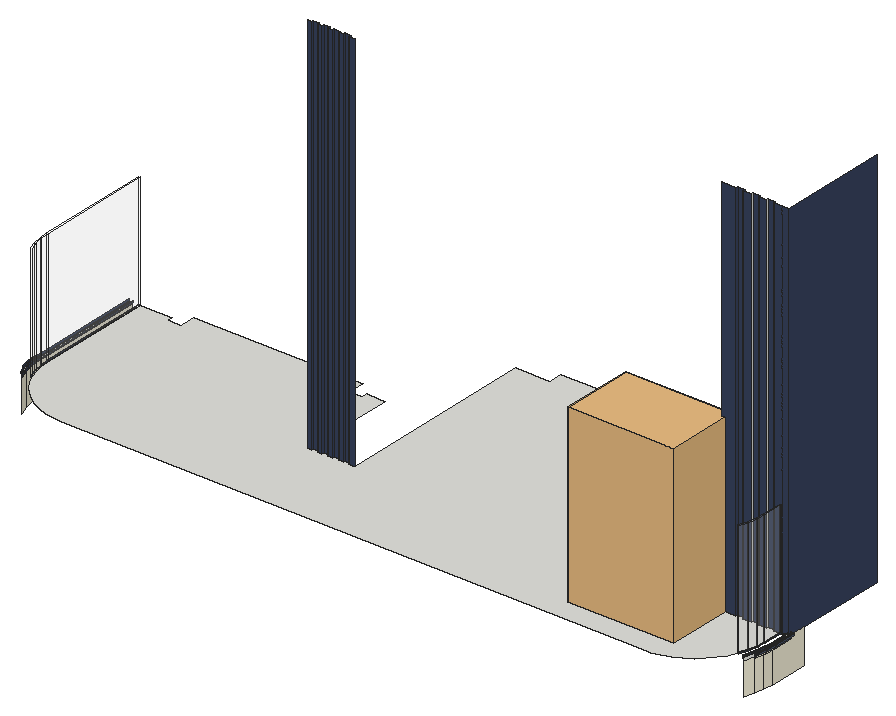
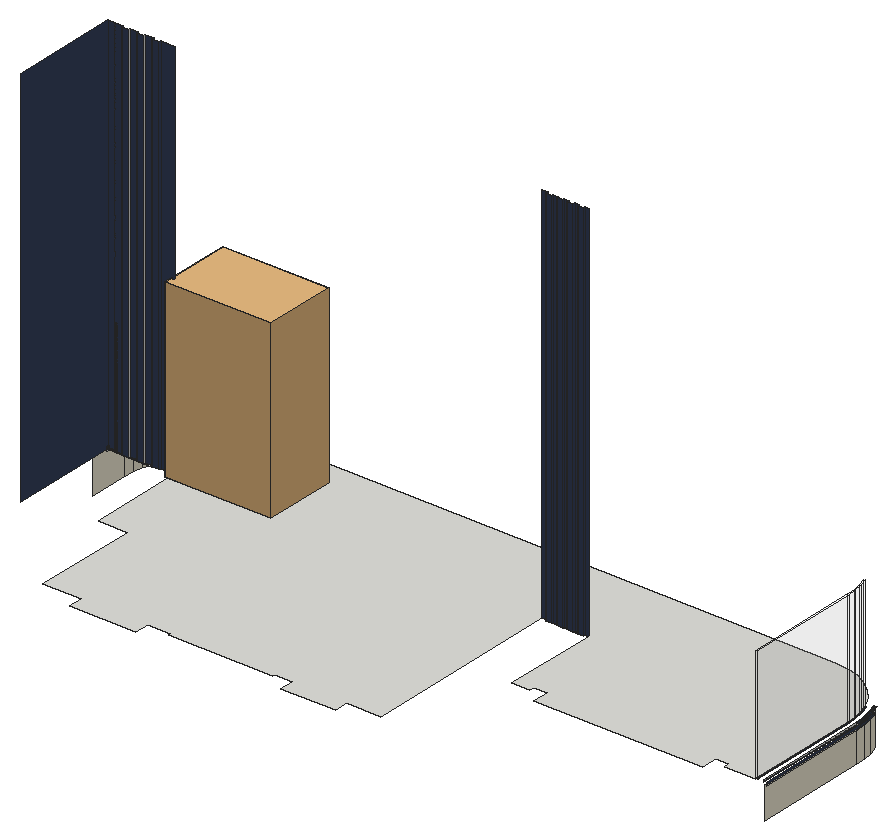
# SketchUp Ruby script. Lengths in inches.
U = 1.inch
M = Sketchup.active_model
def pt(a) = Geom::Point3d.new(a.map { |v| v * U })
def face(e, loops, mat)
  f = e.add_face(loops[0].map { |a| pt(a) })
  loops[1..].each { |l| e.add_face(l.map { |a| pt(a) }).erase! }
  f.material = f.back_material = mat if mat
  f
end
# faces: each face lists its corners as indices into pts; further lists are holes
def faces(e, pts, list, mat = nil) = list.each { |f| face(e, (f[0].is_a?(Array) ? f : [f]).map { |l| l.map { |i| pts[i] } }, mat) }
# xy, xz, yz: faces in a plane at the given z, y or x. An outline is a flat list of corners, or four numbers for a rectangle; further outlines are holes
def ring(l) = l.size == 4 ? [[l[0], l[1]], [l[2], l[1]], [l[2], l[3]], [l[0], l[3]]] : l.each_slice(2).to_a
def flat(e, list, mat, &to3) = list.each { |f| face(e, (f[0].is_a?(Array) ? f : [f]).map { |l| ring(l).map { |u, v| to3.(u, v) } }, mat) }
def xy(e, z, list, mat = nil) = flat(e, list, mat) { |x, y| [x, y, z] }
def xz(e, y, list, mat = nil) = flat(e, list, mat) { |x, z| [x, y, z] }
def yz(e, x, list, mat = nil) = flat(e, list, mat) { |y, z| [x, y, z] }
def lines(e, pts, list) = list.each { |a, b| e.add_line(pt(pts[a]), pt(pts[b])) }
# prism: a flat outline (further loops are holes) pulled along v
def prism(e, loops, v, mat = nil)
  f = face(e, loops, mat); d = Geom::Vector3d.new(v.map { |x| x * U })
  f.pushpull(f.normal.samedirection?(d) ? d.length : -d.length)
end
def box(e, o, s, mat = nil) = prism(e, [[o, [o[0] + s[0], o[1], o[2]], [o[0] + s[0], o[1] + s[1], o[2]], [o[0], o[1] + s[1], o[2]]]], [0, 0, s[2]], mat)
def at(x, y, z, deg = 0) = Geom::Transformation.translation(pt([x, y, z])) * Geom::Transformation.rotation(ORIGIN, Z_AXIS, deg.degrees)
def axes(o, x, y, z) = Geom::Transformation.new([*x, 0, *y, 0, *z, 0, *pt(o).to_a, 1])
def part(name) = M.definitions.add(name)
# library, detail: a bought-in or finely detailed component or shape, given as its bounding box
def library(name, o, s) = part(name).tap { |d| box(d.entities, o, s) }
def detail(e, o, s) = box(e.add_group.entities, o, s)
def put(e, d, t, mat = nil) = e.add_instance(d, t).tap { |i| i.material = mat if mat }
def group(e, t, mat = nil) = e.add_group.tap { |g| g.transformation = t; g.material = mat if mat }.entities
root = M.entities
M.materials.add("0344 AP 9635 Ganges Midnight-N").color = [69, 80, 105]
M.materials.add("0360 AP 9644 Monsoon Midnight-N").color = [56, 67, 95]
M.materials.add("0905 AP 7844 MILD YELLOW").color = [242, 237, 215]
M.materials.add("Glass Clear 001").color = [246, 246, 246]
M.materials["Glass Clear 001"].alpha = 0.1
c1 = library("Ficus triangularis Variegata 002",[-17,-11.8,0.01],[33.04,22.7,54.61])
xy(root,132,[[57,32.69,238.5625,32.69,241.34,32.87,244.0625,33.41,246.69,34.31,249.1875,35.54,251.5,37.08,253.59,38.91,255.42,41,256.96,43.3125,258.19,45.81,259.09,48.4375,259.63,51.16,259.81,53.9375,259.81,60.0625,257.875,60.0625,257.875,60.55,255.6875,60.55,255.6875,60.0625,253.125,60.0625,253.125,60.55,250.9375,60.55,250.9375,60.0625,248.375,60.0625,248.375,60.55,246.1875,60.55,246.1875,60.0625,241.5625,60.0625,241.5625,89.9375,232.5625,89.9375,232.5625,122.9375,220.5625,122.9375,220.5625,127.4375,199.92,127.4375,199.92,122.9375,192.74,122.9375,192.74,123.43,160.18,123.43,160.18,122.9375,154.56,122.9375,154.56,127.4375,137.54,127.4375,137.54,122.9375,126.8125,122.9375,126.8125,60.0625,125.0625,60.0625,125.0625,60.55,123.25,60.55,123.25,60.0625,121.75,60.0625,121.75,60.55,119.9375,60.55,119.9375,60.0625,118.4375,60.0625,118.4375,60.55,116.625,60.55,116.625,60.0625,115.125,60.0625,115.125,60.55,113.3125,60.55,113.3125,60.0625,112.1875,60.0625,112.1875,89.9375,106.59,89.9375,106.59,88.375,102.41,88.375,102.41,93.58,49.72,93.58,49.72,88.375,45.54,88.375,45.54,89.9375,35.75,89.9375,35.75,53.9375,35.94,51.16,36.48,48.4375,37.37,45.81,38.6,43.3125,40.14,41,41.98,38.91,44.07,37.08,46.375,35.54,48.87,34.31,51.5,33.41,54.23,32.87],[115.125,60.0625,116.625,60.55],[118.4375,60.0625,119.9375,60.55],[121.75,60.0625,123.25,60.55],[248.375,60.0625,250.9375,60.55],
  [253.125,60.0625,255.6875,60.55],[257.875,60.0625,262.21,60.55],[262.21,60.0625,262.5625,60.55],[262.21,60.55,262.5625,60.91]])
xz(root,60.0625,[[259.81,132,260.1875,168],[262.21,132,262.5625,132.625]])
xz(root,60.0625,[[112.1875,132,113.3125,252],[115.125,132,116.625,252],[118.4375,132,119.9375,252],[121.75,132,123.25,252],[125.0625,132,126.8125,252],
  [241.5625,132,246.1875,252],[248.375,132,250.9375,252],[253.125,132,255.6875,252],[257.875,132,259.81,132,259.81,168.3125,260.1875,168.3125,260.1875,132.1875,260.4375,132.1875,260.4375,252,257.875,252],[260.1875,132,260.4375,132.1875],
  [260.4375,132,262.21,132.1875],[262.5625,132,262.625,252],[260.4375,132.1875,262.21,132.1875,262.21,132.8125,262.5625,132.8125,262.5625,252,260.4375,252],[262.21,132.625,262.5625,132.8125]],"0360 AP 9644 Monsoon Midnight-N")
xz(root,60.47,[[262.48,132.5625,262.5625,132.625]])
xz(root,60.47,[[262.48,132.625,262.5625,132.8125],[262.5625,132.625,262.97,132.8125]],"0360 AP 9644 Monsoon Midnight-N")
xz(root,60.55,[[262.5625,131.3125,263.05,132],[262.5625,132,263.05,132.625]])
xz(root,60.55,[[113.3125,132,115.125,252],[116.625,132,118.4375,252],[119.9375,132,121.75,252],[123.25,132,125.0625,252],[246.1875,132,248.375,252],
  [250.9375,132,253.125,252],[255.6875,132,257.875,252],[262.5625,132.625,263.05,132.8125]],"0360 AP 9644 Monsoon Midnight-N")
xz(root,60.91,[[262.5625,132,263.41,132.5625],[262.5625,132.5625,263.41,132.625]])
xz(root,60.91,[[262.5625,132.625,263.41,132.8125]],"0360 AP 9644 Monsoon Midnight-N")
xz(root,60.99,[[262.48,132.5625,263.49,132.625]])
xz(root,60.99,[[262.48,132.625,263.49,132.8125]],"0360 AP 9644 Monsoon Midnight-N")
yz(root,32.15,[[53.9375,132,89.9375,132.5625]],"0360 AP 9644 Monsoon Midnight-N")
yz(root,32.51,[[53.9375,131.3125,89.9375,132]],"0905 AP 7844 MILD YELLOW")
yz(root,33,[[53.9375,121.25,89.9375,131.3125]],"0905 AP 7844 MILD YELLOW")
yz(root,33.35,[[53.9375,132.1875,89.9375,132.625]])
yz(root,33.35,[[53.9375,132,89.9375,132.1875]],"0360 AP 9644 Monsoon Midnight-N")
yz(root,35.375,[[53.9375,132,89.9375,132.1875]],"0360 AP 9644 Monsoon Midnight-N")
yz(root,35.375,[[53.9375,132.1875,89.9375,168]],"Glass Clear 001")
yz(root,35.75,[[53.9375,132,89.9375,168]],"Glass Clear 001")
yz(root,113.3125,[[60.0625,132,60.55,252]],"0360 AP 9644 Monsoon Midnight-N")
yz(root,115.125,[[60.0625,132,60.55,252]],"0360 AP 9644 Monsoon Midnight-N")
yz(root,116.625,[[60.0625,132,60.55,252]],"0360 AP 9644 Monsoon Midnight-N")
yz(root,118.4375,[[60.0625,132,60.55,252]],"0360 AP 9644 Monsoon Midnight-N")
yz(root,119.9375,[[60.0625,132,60.55,252]],"0360 AP 9644 Monsoon Midnight-N")
yz(root,121.75,[[60.0625,132,60.55,252]],"0360 AP 9644 Monsoon Midnight-N")
yz(root,123.25,[[60.0625,132,60.55,252]],"0360 AP 9644 Monsoon Midnight-N")
yz(root,125.0625,[[60.0625,132,60.55,252]],"0360 AP 9644 Monsoon Midnight-N")
yz(root,246.1875,[[60.0625,132,60.55,252]],"0360 AP 9644 Monsoon Midnight-N")
yz(root,248.375,[[60.0625,132,60.55,252]],"0360 AP 9644 Monsoon Midnight-N")
yz(root,250.9375,[[60.0625,132,60.55,252]])
yz(root,253.125,[[60.0625,132,60.55,252]],"0360 AP 9644 Monsoon Midnight-N")
yz(root,255.6875,[[60.0625,132,60.55,252]])
yz(root,257.875,[[60.0625,132,60.55,252]],"0360 AP 9644 Monsoon Midnight-N")
yz(root,259.81,[[53.9375,132,60.0625,168]],"Glass Clear 001")
yz(root,260.1875,[[53.9375,132,60.0625,132.1875]],"0360 AP 9644 Monsoon Midnight-N")
yz(root,260.1875,[[53.9375,132.1875,60.0625,168]],"Glass Clear 001")
yz(root,262.21,[[53.9375,132,60.0625,132.1875],[53.9375,132.1875,60.0625,132.625],[53.9375,132.625,60.0625,132.8125]],"0360 AP 9644 Monsoon Midnight-N")
yz(root,262.48,[[60.47,132.5625,60.99,132.625]])
yz(root,262.48,[[60.47,132.625,60.99,132.8125]],"0360 AP 9644 Monsoon Midnight-N")
yz(root,262.5625,[[53.9375,131.3125,60.0625,132.625],[60.0625,131.3125,60.55,132],[60.0625,132,60.55,132,60.55,132.5625,60.47,132.5625,60.47,132.625,60.0625,132.625],[60.55,132,60.91,132.5625],[60.47,132.5625,60.55,132.625],
  [60.55,132.5625,60.91,132.625]])
yz(root,262.5625,[[60.91,132,94.4375,132,94.4375,252,60.0625,252,60.0625,132.8125,60.91,132.8125],[53.9375,132.625,60.0625,132.8125],[60.0625,132.625,60.47,132.8125],[60.47,132.625,60.55,132.8125],[60.55,132.625,60.91,132.8125]],"0360 AP 9644 Monsoon Midnight-N")
yz(root,262.5625,[[53.9375,121.25,65.9375,121.25,65.9375,132,60.55,132,60.55,131.3125,53.9375,131.3125]],"0905 AP 7844 MILD YELLOW")
yz(root,262.97,[[53.9375,132.625,60.47,132.8125]],"0360 AP 9644 Monsoon Midnight-N")
yz(root,263.05,[[53.9375,132,60.55,132.625]])
yz(root,263.05,[[53.9375,131.3125,60.55,132]],"0344 AP 9635 Ganges Midnight-N")
yz(root,263.05,[[53.9375,132.625,60.55,132.8125]],"0360 AP 9644 Monsoon Midnight-N")
yz(root,263.41,[[53.9375,132.5625,60.91,132.625]])
yz(root,263.41,[[53.9375,132,60.91,132.5625]],"0344 AP 9635 Ganges Midnight-N")
yz(root,263.41,[[53.9375,132.625,60.91,132.8125]],"0360 AP 9644 Monsoon Midnight-N")
yz(root,263.49,[[53.9375,132.5625,60.99,132.625],[53.9375,132.625,60.99,132.8125]],"0360 AP 9644 Monsoon Midnight-N")
p = [[34.83,44.75,121.25],[34.83,44.75,131.3125],[33.82,47.73,131.3125],[33.82,47.73,121.25],[261.74,47.73,121.25],[261.74,47.73,131.3125],
  [260.74,44.75,131.3125],[260.74,44.75,121.25],[33.21,50.8,131.3125],[33.21,50.8,121.25],[262.36,50.8,121.25],[262.36,50.8,131.3125],
  [33,53.9375,131.3125],[33,53.9375,121.25],[262.5625,53.9375,121.25],[262.5625,53.9375,131.3125],[34.83,44.75,132.625],[33.82,47.73,132.625],
  [261.74,47.73,132.625],[260.74,44.75,132.625],[33.34,47.6,132],[32.72,50.74,132],[32.72,50.74,131.3125],[33.34,47.6,131.3125],
  [262.85,50.74,132],[262.22,47.6,132],[262.22,47.6,131.3125],[262.85,50.74,131.3125],[33.21,50.8,132.625],[262.36,50.8,132.625],
  [32.51,53.9375,132],[32.51,53.9375,131.3125],[263.05,53.9375,132],[263.05,53.9375,131.3125],[33,53.9375,132.625],[262.5625,53.9375,132.625],
  [35.15,44.89,132],[34.16,47.82,132],[34.16,47.82,132.1875],[35.15,44.89,132.1875],[261.4,47.82,132],[260.41,44.89,132],
  [260.41,44.89,132.1875],[261.4,47.82,132.1875],[36.11,48.34,132],[37.02,45.66,132],[37.02,45.66,132.1875],[36.11,48.34,132.1875],
  [258.54,45.66,132],[259.45,48.34,132],[259.45,48.34,132.1875],[258.54,45.66,132.1875],[37.37,45.81,132],[36.48,48.4375,132],
  [36.48,48.4375,168],[37.37,45.81,168],[259.09,48.4375,132],[258.19,45.81,132],[258.19,45.81,168],[259.09,48.4375,168],
  [32.37,50.69,132],[33,47.51,132],[33,47.51,132.5625],[32.37,50.69,132.5625],[262.5625,47.51,132],[263.19,50.69,132],
  [263.19,50.69,132.5625],[262.5625,47.51,132.5625],[32.72,50.74,132.625],[33.34,47.6,132.625],[262.22,47.6,132.625],[262.85,50.74,132.625],
  [33.56,50.85,132],[33.56,50.85,132.1875],[262.01,50.85,132],[262.01,50.85,132.1875],[35.56,51.11,132],[35.56,51.11,132.1875],
  [260,51.11,132],[260,51.11,132.1875],[35.94,51.16,132],[35.94,51.16,168],[259.63,51.16,132],[259.63,51.16,168],
  [32.15,53.9375,132],[32.15,53.9375,132.5625],[32.51,53.9375,132.625],[263.05,53.9375,132.625],[263.41,53.9375,132],[263.41,53.9375,132.5625],
  [33.35,53.9375,132],[33.35,53.9375,132.1875],[262.21,53.9375,132],[262.21,53.9375,132.1875],[35.375,53.9375,132],[35.375,53.9375,132.1875],
  [260.1875,53.9375,132],[260.1875,53.9375,132.1875],[35.75,53.9375,132],[35.75,53.9375,168],[259.81,53.9375,132],[259.81,53.9375,168],
  [35.15,44.89,132.625],[34.16,47.82,132.625],[261.4,47.82,132.625],[260.41,44.89,132.625],[36.11,48.34,168],[37.02,45.66,168],
  [258.54,45.66,168],[259.45,48.34,168],[33.56,50.85,132.625],[262.01,50.85,132.625],[35.56,51.11,168],[260,51.11,168],
  [33.35,53.9375,132.625],[262.21,53.9375,132.625],[35.375,53.9375,168],[260.1875,53.9375,168],[34.45,44.6,132.625],[33.42,47.62,132.625],
  [33.42,47.62,132.8125],[34.45,44.6,132.8125],[262.14,47.62,132.625],[261.12,44.6,132.625],[261.12,44.6,132.8125],[262.14,47.62,132.8125],
  [33.82,47.73,132.8125],[34.83,44.75,132.8125],[260.74,44.75,132.8125],[261.74,47.73,132.8125],[34.16,47.82,132.8125],[35.15,44.89,132.8125],
  [260.41,44.89,132.8125],[261.4,47.82,132.8125],[32.29,50.68,132.5625],[32.92,47.49,132.5625],[32.92,47.49,132.625],[32.29,50.68,132.625],
  [32.92,47.49,132.8125],[32.29,50.68,132.8125],[32.37,50.69,132.625],[33,47.51,132.625],[32.37,50.69,132.8125],[33,47.51,132.8125],
  [262.64,47.49,132.5625],[263.27,50.68,132.5625],[263.27,50.68,132.625],[262.64,47.49,132.625],[263.27,50.68,132.8125],[262.64,47.49,132.8125],
  [262.5625,47.51,132.625],[263.19,50.69,132.625],[262.5625,47.51,132.8125],[263.19,50.69,132.8125],[32.72,50.74,132.8125],[33.34,47.6,132.8125],
  [32.8,50.75,132.625],[32.8,50.75,132.8125],[262.77,50.75,132.625],[262.77,50.75,132.8125],[262.22,47.6,132.8125],[262.85,50.74,132.8125],
  [33.21,50.8,132.8125],[262.36,50.8,132.8125],[33.56,50.85,132.8125],[262.01,50.85,132.8125],[32.07,53.9375,132.5625],[32.07,53.9375,132.625],
  [32.07,53.9375,132.8125],[32.15,53.9375,132.625],[32.15,53.9375,132.8125],[32.51,53.9375,132.8125],[263.05,53.9375,132.8125],[263.41,53.9375,132.625],
  [263.41,53.9375,132.8125],[263.49,53.9375,132.5625],[263.49,53.9375,132.625],[263.49,53.9375,132.8125],[32.59,53.9375,132.625],[32.59,53.9375,132.8125],
  [33,53.9375,132.8125],[262.5625,53.9375,132.8125],[262.97,53.9375,132.625],[262.97,53.9375,132.8125],[33.35,53.9375,132.8125],[262.21,53.9375,132.8125]]
faces(root,p,[[0,1,2,3],[4,5,6,7],[3,2,8,9],[10,11,5,4],[9,8,12,13],[14,15,11,10],[20,21,22,23],[24,25,26,27],
  [21,30,31,22],[32,24,27,33]],"0905 AP 7844 MILD YELLOW")
faces(root,p,[[1,16,17,2],[5,18,19,6],[2,17,28,8],[11,29,18,5],[8,28,34,12],[15,35,29,11],[20,21,68,69],[24,25,70,71],
  [21,30,86,68],[32,24,71,87],[62,63,140,141],[66,67,150,151],[63,85,169,140],[89,66,151,173]])
faces(root,p,[[36,37,38,39],[40,41,42,43],[44,45,46,47],[48,49,50,51],[60,61,62,63],[37,72,73,38],[74,40,43,75],[76,44,47,77],
  [49,78,79,50],[84,60,63,85],[72,90,91,73],[92,74,75,93],[94,76,77,95],[78,96,97,79],[102,39,38,103],[104,43,42,105],
  [103,38,73,110],[111,75,43,104],[110,73,91,114],[115,93,75,111],[118,119,120,121],[122,123,124,125],[16,17,126,127],[18,19,128,129],
  [102,103,130,131],[104,105,132,133],[134,135,136,137],[137,136,138,139],[141,140,142,143],[144,145,146,147],[147,146,148,149],[151,150,152,153],
  [69,68,154,155],[119,156,157,120],[158,122,125,159],[71,70,160,161],[17,28,162,126],[29,18,129,163],[103,110,164,130],[111,104,133,165],
  [166,134,137,167],[167,137,139,168],[140,169,170,142],[68,86,171,154],[87,71,161,172],[173,151,153,174],[145,175,176,146],[146,176,177,148],
  [156,178,179,157],[28,34,180,162],[35,29,163,181],[182,158,159,183],[110,114,184,164],[115,111,165,185]],"0360 AP 9644 Monsoon Midnight-N")
faces(root,p,[[52,53,54,55],[56,57,58,59],[53,80,81,54],[82,56,59,83],[80,98,99,81],[100,82,83,101],[106,47,46,107],[108,51,50,109],
  [112,77,47,106],[109,50,79,113],[116,95,77,112],[113,79,97,117]],"Glass Clear 001")
faces(root,p,[[64,65,66,67],[65,88,89,66]],"0344 AP 9635 Ganges Midnight-N")
put(root,c1,at(226.74,51.64,132))
